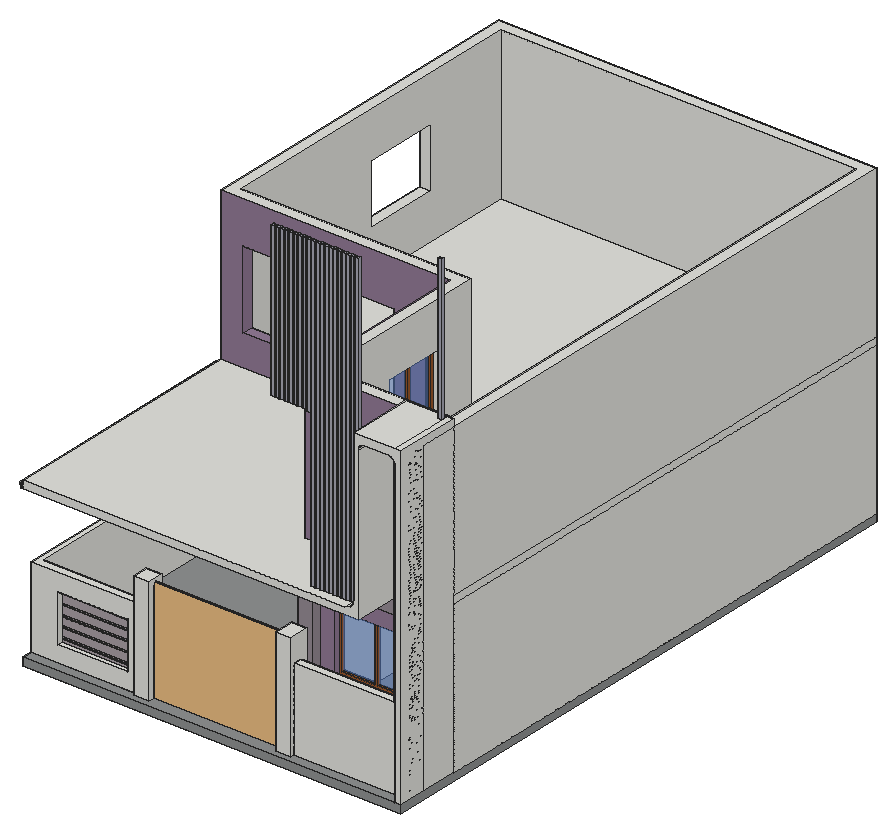
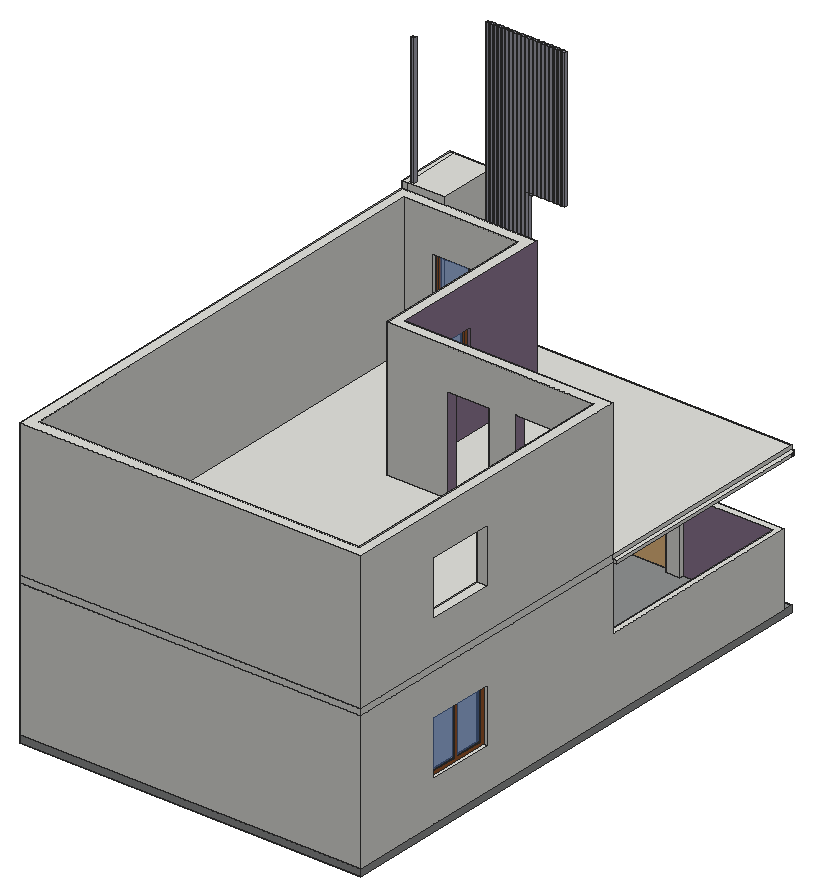
# SketchUp Ruby script. Lengths in inches.
U = 1.inch
M = Sketchup.active_model
def pt(a) = Geom::Point3d.new(a.map { |v| v * U })
def face(e, loops, mat)
  f = e.add_face(loops[0].map { |a| pt(a) })
  loops[1..].each { |l| e.add_face(l.map { |a| pt(a) }).erase! }
  f.material = f.back_material = mat if mat
  f
end
# faces: each face lists its corners as indices into pts; further lists are holes
def faces(e, pts, list, mat = nil) = list.each { |f| face(e, (f[0].is_a?(Array) ? f : [f]).map { |l| l.map { |i| pts[i] } }, mat) }
# xy, xz, yz: faces in a plane at the given z, y or x. An outline is a flat list of corners, or four numbers for a rectangle; further outlines are holes
def ring(l) = l.size == 4 ? [[l[0], l[1]], [l[2], l[1]], [l[2], l[3]], [l[0], l[3]]] : l.each_slice(2).to_a
def flat(e, list, mat, &to3) = list.each { |f| face(e, (f[0].is_a?(Array) ? f : [f]).map { |l| ring(l).map { |u, v| to3.(u, v) } }, mat) }
def xy(e, z, list, mat = nil) = flat(e, list, mat) { |x, y| [x, y, z] }
def xz(e, y, list, mat = nil) = flat(e, list, mat) { |x, z| [x, y, z] }
def yz(e, x, list, mat = nil) = flat(e, list, mat) { |y, z| [x, y, z] }
def lines(e, pts, list) = list.each { |a, b| e.add_line(pt(pts[a]), pt(pts[b])) }
# prism: a flat outline (further loops are holes) pulled along v
def prism(e, loops, v, mat = nil)
  f = face(e, loops, mat); d = Geom::Vector3d.new(v.map { |x| x * U })
  f.pushpull(f.normal.samedirection?(d) ? d.length : -d.length)
end
def box(e, o, s, mat = nil) = prism(e, [[o, [o[0] + s[0], o[1], o[2]], [o[0] + s[0], o[1] + s[1], o[2]], [o[0], o[1] + s[1], o[2]]]], [0, 0, s[2]], mat)
def at(x, y, z, deg = 0) = Geom::Transformation.translation(pt([x, y, z])) * Geom::Transformation.rotation(ORIGIN, Z_AXIS, deg.degrees)
def axes(o, x, y, z) = Geom::Transformation.new([*x, 0, *y, 0, *z, 0, *pt(o).to_a, 1])
def part(name) = M.definitions.add(name)
# library, detail: a bought-in or finely detailed component or shape, given as its bounding box
def library(name, o, s) = part(name).tap { |d| box(d.entities, o, s) }
def detail(e, o, s) = box(e.add_group.entities, o, s)
def put(e, d, t, mat = nil) = e.add_instance(d, t).tap { |i| i.material = mat if mat }
def group(e, t, mat = nil) = e.add_group.tap { |g| g.transformation = t; g.material = mat if mat }.entities
root = M.entities
M.materials.add("0300 AP 7184 STILL POND").color = [167, 167, 180]
M.materials.add("1349 AP 9111 FRESH ORCHID").color = [145, 122, 149]
M.materials.add("1372 AP K056 Arctic Mauve-N").color = [168, 159, 165]
M.materials.add("1373 AP K057 Mauve Meditation-N").color = [149, 139, 148]
M.materials.add("[Blacktop Old 02]").color = [143, 145, 145]
M.materials.add("[Translucent Glass Blue]").color = [100, 149, 237]
M.materials["[Translucent Glass Blue]"].alpha = 0.5
M.materials.add("[Wood Cherry Original]").color = [152, 86, 42]
c1 = library("Untitled",[0,0,0],[36,4.39,84])
c2 = library("Modern Gate 1",[0,0,0],[118.11,1.97,78.74])
c3 = part("Group\#20")
box(c3.entities,[0,0,0],[3.0625,2.375,246])
c4 = part("Group\#10")
box(c4.entities,[0,0,124.49],[3.0625,2.375,121.51])
c5 = part("Group\#19")
xy(c5.entities,0.11,[[0,0,3.0625,2.375]])
xy(c5.entities,246,[[0,0,3.0625,2.375]])
xz(c5.entities,0,[[0,0.11,3.0625,246]])
xz(c5.entities,2.375,[[0,0.11,3.0625,124.49],[0,124.49,3.0625,246]])
yz(c5.entities,0,[[0,0.11,2.375,124.49],[0,124.49,2.375,246]])
yz(c5.entities,3.0625,[[0,0.11,2.375,246]])
c6 = part("Group10\#2")
xy(c6.entities,0,[[-21.5,-21.5,-1.25,21.5],[1.25,-21.5,21.5,21.5]])
c7 = part("Group9\#1")
prism(c7.entities,[[[24,-24,0],[-24,-24,0],[-24,24,0],[24,24,0]],[[-1.25,21.5,0],[-21.5,21.5,0],[-21.5,-21.5,0],[-1.25,-21.5,0]],[[1.25,-21.5,0],[21.5,-21.5,0],[21.5,21.5,0],[1.25,21.5,0]]],[0,0,2])
put(c7.entities,c6,at(0,0,1),"[Translucent Glass Blue]")
c8 = part("Group12\#2")
xy(c8.entities,0,[[-27.5,-21.5,-1.25,21.5],[1.25,-21.5,27.5,21.5]])
c9 = part("Group11\#2")
prism(c9.entities,[[[-30,24,0],[30,24,0],[30,-24,0],[-30,-24,0]],[[1.25,21.5,0],[1.25,-21.5,0],[27.5,-21.5,0],[27.5,21.5,0]],[[-1.25,-21.5,0],[-1.25,21.5,0],[-27.5,21.5,0],[-27.5,-21.5,0]]],[0,0,2])
put(c9.entities,c8,at(0,0,1),"[Translucent Glass Blue]")
c10 = part("Group9\#2")
prism(c10.entities,[[[24,-24,0],[-24,-24,0],[-24,24,0],[24,24,0]],[[-1.25,21.5,0],[-21.5,21.5,0],[-21.5,-21.5,0],[-1.25,-21.5,0]],[[1.25,-21.5,0],[21.5,-21.5,0],[21.5,21.5,0],[1.25,21.5,0]]],[0,0,2])
put(c10.entities,c6,at(0,0,1),"[Translucent Glass Blue]")
c11 = part("Group11\#1")
prism(c11.entities,[[[-30,24,0],[30,24,0],[30,-24,0],[-30,-24,0]],[[1.25,21.5,0],[1.25,-21.5,0],[27.5,-21.5,0],[27.5,21.5,0]],[[-1.25,-21.5,0],[-1.25,21.5,0],[-27.5,21.5,0],[-27.5,-21.5,0]]],[0,0,2])
put(c11.entities,c8,at(0,0,1),"[Translucent Glass Blue]")
c12 = part("Group63\#2")
xy(c12.entities,0,[[-26.0625,-26.25,-9.48,26.25],[-8.29,-26.25,8.29,26.25],[9.48,-26.25,26.0625,26.25]])
c13 = part("Group62\#1")
prism(c13.entities,[[[-30,-30.1875,0],[-30,30.1875,0],[30,30.1875,0],[30,-30.1875,0]],[[-9.48,26.25,0],[-26.0625,26.25,0],[-26.0625,-26.25,0],[-9.48,-26.25,0]],[[9.48,26.25,0],[9.48,-26.25,0],[26.0625,-26.25,0],[26.0625,26.25,0]],[[-8.29,26.25,0],[-8.29,-26.25,0],[8.29,-26.25,0],[8.29,26.25,0]]],[0,0,5.875])
put(c13.entities,c12,at(0,0,2.9375),"[Translucent Glass Blue]")
c14 = part("Group4\#2")
xy(c14.entities,0,[[-27.5,-21.5,-1.25,21.5],[1.25,-21.5,27.5,21.5]])
c15 = part("Group3\#1")
prism(c15.entities,[[[30,24,0],[30,-24,0],[-30,-24,0],[-30,24,0]],[[27.5,-21.5,0],[27.5,21.5,0],[1.25,21.5,0],[1.25,-21.5,0]],[[-27.5,21.5,0],[-27.5,-21.5,0],[-1.25,-21.5,0],[-1.25,21.5,0]]],[0,0,2])
put(c15.entities,c14,at(0,0,1),"[Translucent Glass Blue]")
g1 = group(root,at(21.875,58.1875,-6),"[Blacktop Old 02]")
box(g1,[0,-52.5625,0],[300,472.5625,6])
put(root,c1,at(123.5625,204.4,0))
put(root,c2,axes([117.75,16.2,0],[0.83803,0,0],[0,1,0],[0,0,1.0465]))
g2 = group(root,at(21.875,58.1875,120))
xy(g2,-120,[[295.5,-52.5625,300,-29.9375]])
xy(g2,0,[[0.83,-52.5625,-0.63,-52.43,-1.82,-52.03,-2.75,-51.37,-3.41,-50.44,-3.81,-49.25,-3.9375,-47.8,-3.9375,144.125,0,144.125,0,420,300,420,300,0,266.53,0,266.53,-52.5625]])
xy(g2,3,[[0,-52.5625,0,144.125,-3.9375,144.125,-3.9375,-47.8,-3.83,-49.25,-3.5,-50.44,-2.95,-51.37,-2.1875,-52.03,-1.2,-52.43]])
xy(g2,6,[[0,-52.5625,255.76,-52.5625,255.76,0,300,0,300,420,0,420]])
xy(g2,126,[[271.39,-52.5625,271.39,0,295.5,0,295.5,-29.9375,288.53,-29.9375,288.53,-52.5625],[295.5,-29.9375,300,0]])
xy(g2,132,[[262.58,-52.5625,295.5,0],[295.5,-52.5625,300,0]])
xz(g2,-52.5625,[[295.5,-120,300,-120,300,132,262.58,132,262.58,12.82,262.39,10.74,261.82,9.03,260.875,7.7,259.55,6.76,257.84,6.1875,255.76,6,0,6,0,3,0.83,0,266.53,0,266.53,121.14,266.67,122.625,267.07,123.84,267.75,124.78,268.69,125.46,269.91,125.86,271.39,126,288.53,126,290.66,125.81,292.4,125.23,293.76,124.26,294.73,122.9,295.31,121.16,295.5,119.03]])
xz(g2,-29.9375,[[295.5,-120,295.5,119.03,295.31,121.16,294.73,122.9,293.76,124.26,292.4,125.23,290.66,125.81,288.53,126,300,126,300,-120]])
xz(g2,0,[[266.53,0,300,6],[255.76,6,257.84,6.1875,259.55,6.76,260.875,7.7,261.82,9.03,262.39,10.74,262.58,12.82,262.58,132,295.5,132,295.5,126,271.39,126,269.91,125.86,268.69,125.46,267.75,124.78,267.07,123.84,266.67,122.625,266.53,121.14,266.53,6],[295.5,126,300,132]])
xz(g2,144.125,[[-3.9375,0,0,3]])
xz(g2,420,[[0,0,300,6]])
yz(g2,-3.9375,[[-47.8,0,144.125,3]])
yz(g2,0,[[144.125,0,420,6],[-52.5625,3,144.125,6]])
yz(g2,262.58,[[-52.5625,12.82,0,132]])
yz(g2,266.53,[[-52.5625,0,0,121.14]])
yz(g2,295.5,[[-52.5625,-120,-29.9375,119.03]])
yz(g2,300,[[-52.5625,-120,-29.9375,-120,-29.9375,126,0,126,0,132,-52.5625,132],[0,0,420,6]])
p = [[-0.63,-52.43,0],[0.83,-52.5625,0],[-1.2,-52.43,3],[0,-52.5625,3],[-2.1875,-52.03,3],[-1.82,-52.03,0],
  [-2.95,-51.37,3],[-2.75,-51.37,0],[-3.5,-50.44,3],[-3.41,-50.44,0],[-3.81,-49.25,0],[-3.83,-49.25,3],
  [-3.9375,-47.8,3],[-3.9375,-47.8,0],[257.84,-52.5625,6.1875],[257.84,0,6.1875],[255.76,0,6],[255.76,-52.5625,6],
  [259.55,-52.5625,6.76],[259.55,0,6.76],[260.875,-52.5625,7.7],[260.875,0,7.7],[261.82,-52.5625,9.03],[261.82,0,9.03],
  [262.39,-52.5625,10.74],[262.39,0,10.74],[262.58,-52.5625,12.82],[262.58,0,12.82],[295.31,-52.5625,121.16],[295.31,-29.9375,121.16],
  [295.5,-29.9375,119.03],[295.5,-52.5625,119.03],[266.67,0,122.625],[266.67,-52.5625,122.625],[266.53,-52.5625,121.14],[266.53,0,121.14],
  [294.73,-52.5625,122.9],[294.73,-29.9375,122.9],[267.07,0,123.84],[267.07,-52.5625,123.84],[293.76,-52.5625,124.26],[293.76,-29.9375,124.26],
  [267.75,0,124.78],[267.75,-52.5625,124.78],[292.4,-52.5625,125.23],[292.4,-29.9375,125.23],[268.69,0,125.46],[268.69,-52.5625,125.46],
  [290.66,-52.5625,125.81],[290.66,-29.9375,125.81],[269.91,0,125.86],[269.91,-52.5625,125.86],[288.53,-52.5625,126],[288.53,-29.9375,126],
  [271.39,0,126],[271.39,-52.5625,126]]
faces(g2,p,[[0,1,2],[1,3,2],[0,2,4],[5,0,4],[5,4,6],[7,5,6],[7,6,8],[9,7,8],
  [10,9,11],[9,8,11],[10,11,12],[13,10,12],[14,15,16,17],[18,19,15,14],[20,21,19,18],[22,23,21,20],
  [24,25,23,22],[26,27,25,24],[28,29,30,31],[32,33,34,35],[36,37,29,28],[38,39,33,32],[40,41,37,36],[42,43,39,38],
  [44,45,41,40],[46,47,43,42],[48,49,45,44],[50,51,47,46],[52,53,49,48],[54,55,51,50]])
put(g2,c3,at(226.96,-45.3125,6),"0300 AP 7184 STILL POND")
g3 = group(g2,at(230.4,-45.3125,6),"0300 AP 7184 STILL POND")
box(g3,[0,0,0],[3.0625,2.375,246])
put(g2,c3,at(233.84,-45.3125,6),"0300 AP 7184 STILL POND")
put(g2,c3,at(237.28,-45.3125,6),"0300 AP 7184 STILL POND")
put(g2,c3,at(240.71,-45.3125,6),"0300 AP 7184 STILL POND")
put(g2,c3,at(244.15,-45.3125,6),"0300 AP 7184 STILL POND")
put(g2,c3,at(247.59,-45.3125,6),"0300 AP 7184 STILL POND")
put(g2,c3,at(251.03,-45.3125,6),"0300 AP 7184 STILL POND")
put(g2,c3,at(254.46,-45.3125,6),"0300 AP 7184 STILL POND")
put(g2,c3,at(257.9,-45.3125,6),"0300 AP 7184 STILL POND")
put(g2,c4,at(191.3125,-45.3125,6),"0300 AP 7184 STILL POND")
put(g2,c4,at(194.89,-45.3125,6),"0300 AP 7184 STILL POND")
put(g2,c4,at(198.46,-45.3125,6),"0300 AP 7184 STILL POND")
put(g2,c4,at(202.04,-45.3125,6),"0300 AP 7184 STILL POND")
put(g2,c4,at(205.61,-45.3125,6),"0300 AP 7184 STILL POND")
put(g2,c4,at(209.1875,-45.3125,6),"0300 AP 7184 STILL POND")
put(g2,c4,at(212.76,-45.3125,6),"0300 AP 7184 STILL POND")
put(g2,c4,at(216.33,-45.3125,6),"0300 AP 7184 STILL POND")
g4 = group(g2,at(219.96,-45.3125,6),"0300 AP 7184 STILL POND")
xy(g4,123.23,[[0,0,3.0625,2.375]])
xy(g4,246,[[0,0,3.0625,2.375]])
xz(g4,0,[[0,123.23,3.0625,246]])
xz(g4,2.375,[[0,123.23,3.0625,124.49],[0,124.49,3.0625,246]])
yz(g4,0,[[0,123.23,2.375,124.49],[0,124.49,2.375,246]])
yz(g4,3.0625,[[0,123.23,2.375,246]])
put(g2,c5,at(223.24,-45.3125,5.89),"0300 AP 7184 STILL POND")
g5 = group(g2,at(267.59,-5.2,-0.11),"0300 AP 7184 STILL POND")
xy(g5,0.11,[[0,0,3.0625,2.375]])
xy(g5,126.11,[[0,0,3.0625,2.375]])
xz(g5,0,[[0,0.11,3.0625,126.11]])
xz(g5,2.375,[[0,0.11,3.0625,124.49],[0,124.49,3.0625,126.11]])
yz(g5,0,[[0,0.11,2.375,124.49],[0,124.49,2.375,126.11]])
yz(g5,3.0625,[[0,0.11,2.375,126.11]])
g6 = group(g2,at(271.03,-5.2,-0.11),"0300 AP 7184 STILL POND")
xy(g6,0.11,[[0,0,3.0625,2.375]])
xy(g6,126.11,[[0,0,3.0625,2.375]])
xz(g6,0,[[0,0.11,3.0625,126.11]])
xz(g6,2.375,[[0,0.11,3.0625,124.49],[0,124.49,3.0625,126.11]])
yz(g6,0,[[0,0.11,2.375,124.49],[0,124.49,2.375,126.11]])
yz(g6,3.0625,[[0,0.11,2.375,126.11]])
g7 = group(g2,at(274.48,-5.2,-0.11),"0300 AP 7184 STILL POND")
xy(g7,0.11,[[0,0,3.0625,2.375]])
xy(g7,126.11,[[0,0,3.0625,2.375]])
xz(g7,0,[[0,0.11,3.0625,126.11]])
xz(g7,2.375,[[0,0.11,3.0625,124.49],[0,124.49,3.0625,126.11]])
yz(g7,0,[[0,0.11,2.375,124.49],[0,124.49,2.375,126.11]])
yz(g7,3.0625,[[0,0.11,2.375,126.11]])
g8 = group(g2,at(277.93,-5.2,-0.11),"0300 AP 7184 STILL POND")
xy(g8,0.11,[[0,0,3.0625,2.375]])
xy(g8,130.6875,[[0,0,3.0625,2.375]])
xz(g8,0,[[0,0.11,3.0625,130.6875]])
xz(g8,2.375,[[0,0.11,3.0625,124.49],[0,124.49,3.0625,130.6875]])
yz(g8,0,[[0,0.11,2.375,124.49],[0,124.49,2.375,130.6875]])
yz(g8,3.0625,[[0,0.11,2.375,130.6875]])
g9 = group(g2,at(281.37,-5.2,-0.11),"0300 AP 7184 STILL POND")
xy(g9,0.11,[[0,0,3.0625,2.375]])
xy(g9,126.01,[[0,0,3.0625,2.375]])
xz(g9,0,[[0,0.11,3.0625,126.01]])
xz(g9,2.375,[[0,0.11,3.0625,124.49],[0,124.49,3.0625,126.01]])
yz(g9,0,[[0,0.11,2.375,124.49],[0,124.49,2.375,126.01]])
yz(g9,3.0625,[[0,0.11,2.375,126.01]])
g10 = group(g2,at(284.82,-5.2,-0.11),"0300 AP 7184 STILL POND")
xy(g10,0.11,[[0,0,3.0625,2.375]])
xy(g10,126.01,[[0,0,3.0625,2.375]])
xz(g10,0,[[0,0.11,3.0625,126.01]])
xz(g10,2.375,[[0,0.11,3.0625,124.49],[0,124.49,3.0625,126.01]])
yz(g10,0,[[0,0.11,2.375,124.49],[0,124.49,2.375,126.01]])
yz(g10,3.0625,[[0,0.11,2.375,126.01]])
g11 = group(g2,at(288.27,-5.2,-0.11),"0300 AP 7184 STILL POND")
xy(g11,0.11,[[0,0,3.0625,2.375]])
xy(g11,126.01,[[0,0,3.0625,2.375]])
xz(g11,0,[[0,0.11,3.0625,126.01]])
xz(g11,2.375,[[0,0.11,3.0625,124.49],[0,124.49,3.0625,126.01]])
yz(g11,0,[[0,0.11,2.375,124.49],[0,124.49,2.375,126.01]])
yz(g11,3.0625,[[0,0.11,2.375,126.01]])
put(g2,c5,at(291.71,-5.2,-0.11),"0300 AP 7184 STILL POND")
g12 = group(root,at(21.875,58.1875,126))
xy(g12,-126,[[196.875,-47.1875,208.875,-31.8125],[208.875,-44.1875,208.875,-37.8125,295,-37.8125,295,-25.4375,300,-25.4375,300,-44.1875],[295,-25.4375,300,0]])
xy(g12,-60.49,[[208.875,-44.1875,288.125,-37.8125]])
xy(g12,-41.05,[[196.875,-47.1875,208.875,-31.8125]])
xy(g12,0,[[182.15,0,182.15,144.125,137.6875,144.125,137.6875,153.125,191.15,153.125,191.15,9,291,9,291,411,9,411,9,153.125,101.6875,153.125,101.6875,144.125,0,144.125,0,420,300,420,300,0]])
xy(g12,24.375,[[17.6875,144.125,77.6875,153.125]],"1349 AP 9111 FRESH ORCHID")
xy(g12,36,[[206.15,4.5,266.15,9],[186.65,72.125,191.15,120.125],[0,281.375,9,341.375]])
xy(g12,36,[[206.15,0,266.15,4.5],[182.15,72.125,186.65,120.125]],"1349 AP 9111 FRESH ORCHID")
xy(g12,84,[[206.15,4.5,266.15,9],[186.65,72.125,191.15,120.125],[0,281.375,9,341.375]])
xy(g12,84,[[206.15,0,266.15,4.5],[182.15,72.125,186.65,120.125],[101.6875,144.125,137.6875,153.125]],"1349 AP 9111 FRESH ORCHID")
xy(g12,86.75,[[17.6875,144.125,77.6875,153.125]],"1349 AP 9111 FRESH ORCHID")
xy(g12,120,[[288.125,-44.1875,300,-44.1875,300,-25.4375,295,-25.4375,295,-37.8125,288.125,-37.8125],[295,-25.4375,300,0],[[182.15,0,300,0,300,420,0,420,0,144.125,182.15,144.125],[191.15,9,191.15,153.125,9,153.125,9,411,291,411,291,9]]])
xz(g12,-47.1875,[[196.875,-126,208.875,-41.05]])
xz(g12,-44.1875,[[208.875,-126,300,-126,300,120,288.125,120,288.125,-60.49,208.875,-60.49]])
xz(g12,-37.8125,[[208.875,-126,208.875,-60.49,288.125,-60.49,288.125,120,295,120,295,-126]])
xz(g12,-31.8125,[[196.875,-126,208.875,-41.05]])
xz(g12,0,[[295,-126,300,0],[295,0,300,120]])
xz(g12,0,[[[182.15,0,295,120],[206.15,36,266.15,84]]],"1349 AP 9111 FRESH ORCHID")
xz(g12,9,[[[191.15,0,291,120],[206.15,36,266.15,84]]])
xz(g12,72.125,[[186.65,36,191.15,84]])
xz(g12,72.125,[[182.15,36,186.65,84]],"1349 AP 9111 FRESH ORCHID")
xz(g12,120.125,[[186.65,36,191.15,84]])
xz(g12,120.125,[[182.15,36,186.65,84]],"1349 AP 9111 FRESH ORCHID")
xz(g12,144.125,[[[0,0,101.6875,0,101.6875,84,137.6875,84,137.6875,0,182.15,0,182.15,120,0,120],[17.6875,24.375,77.6875,86.75]]],"1349 AP 9111 FRESH ORCHID")
xz(g12,153.125,[[[9,0,9,120,191.15,120,191.15,0,137.6875,0,137.6875,84,101.6875,84,101.6875,0],[17.6875,24.375,77.6875,86.75]]])
xz(g12,281.375,[[0,36,9,84]])
xz(g12,341.375,[[0,36,9,84]])
xz(g12,411,[[9,0,291,120]])
xz(g12,420,[[0,0,300,120]])
yz(g12,0,[[[144.125,0,420,120],[281.375,36,341.375,84]]])
yz(g12,9,[[[153.125,0,411,120],[281.375,36,341.375,84]]])
yz(g12,17.6875,[[144.125,24.375,153.125,86.75]],"1349 AP 9111 FRESH ORCHID")
yz(g12,77.6875,[[144.125,24.375,153.125,86.75]],"1349 AP 9111 FRESH ORCHID")
yz(g12,101.6875,[[144.125,0,153.125,84]],"1349 AP 9111 FRESH ORCHID")
yz(g12,137.6875,[[144.125,0,153.125,84]],"1349 AP 9111 FRESH ORCHID")
yz(g12,182.15,[[[0,0,144.125,120],[72.125,36,120.125,84]]],"1349 AP 9111 FRESH ORCHID")
yz(g12,191.15,[[[9,0,153.125,120],[72.125,36,120.125,84]]])
yz(g12,196.875,[[-47.1875,-126,-31.8125,-41.05]])
yz(g12,206.15,[[4.5,36,9,84]])
yz(g12,206.15,[[0,36,4.5,84]],"1349 AP 9111 FRESH ORCHID")
yz(g12,208.875,[[-47.1875,-126,-44.1875,-126,-44.1875,-60.49,-37.8125,-60.49,-37.8125,-126,-31.8125,-126,-31.8125,-41.05,-47.1875,-41.05],[-44.1875,-126,-37.8125,-60.49]])
yz(g12,266.15,[[4.5,36,9,84]])
yz(g12,266.15,[[0,36,4.5,84]],"1349 AP 9111 FRESH ORCHID")
yz(g12,288.125,[[-44.1875,-60.49,-37.8125,120]])
yz(g12,291,[[9,0,411,120]])
yz(g12,295,[[-37.8125,-126,0,120]])
yz(g12,300,[[-44.1875,-126,0,120],[0,0,420,120]])
put(g12,c7,axes([187.65,96.125,60],[0,-1,0],[0,0,1],[-1,0,0]),"[Wood Cherry Original]")
put(g12,c9,axes([236.15,3.5,60],[-1,0,0],[0,0,1],[0,1,0]),"[Wood Cherry Original]")
g13 = group(root,at(21.875,58.1875,0))
xy(g13,0,[[83.875,-47.1875,95.875,-34.8125],[0,-44.1875,83.875,-37.8125],[0,-37.8125,0,420,300,420,300,0,182.15,0,182.15,144.125,137.6875,144.125,137.6875,153.125,191.15,153.125,191.15,9,291,9,291,411,9,411,9,153.125,101.6875,153.125,101.6875,144.125,4.5,144.125,4.5,-37.8125]])
xy(g13,12.64,[[21.17,-44.1875,76.73,-40.3125]])
xy(g13,15.05,[[21.17,-40.3125,76.73,-39.3125]])
xy(g13,16.99,[[21.17,-40.3125,76.73,-39.3125]])
xy(g13,23.05,[[21.17,-40.3125,76.73,-39.3125]])
xy(g13,23.625,[[17.6875,148.625,77.6875,153.125]])
xy(g13,23.625,[[17.6875,144.125,77.6875,148.625]],"1349 AP 9111 FRESH ORCHID")
xy(g13,24.99,[[21.17,-40.3125,76.73,-39.3125]])
xy(g13,31.05,[[21.17,-40.3125,76.73,-39.3125]])
xy(g13,32.99,[[21.17,-40.3125,76.73,-39.3125]])
xy(g13,36,[[0,281.375,4.5,341.375],[4.5,281.375,9,341.375]])
xy(g13,36,[[206.15,0,266.15,4.5],[206.15,4.5,266.15,9],[182.15,72.125,186.65,120.125],[186.65,72.125,191.15,120.125]],"1349 AP 9111 FRESH ORCHID")
xy(g13,39.05,[[21.17,-40.3125,76.73,-39.3125]])
xy(g13,40.99,[[21.17,-40.3125,76.73,-39.3125]])
xy(g13,47.05,[[21.17,-40.3125,76.73,-39.3125]])
xy(g13,48.99,[[21.17,-40.3125,76.73,-39.3125]])
xy(g13,50.58,[[21.17,-44.1875,76.73,-40.3125]])
xy(g13,64.1875,[[0,-44.1875,83.875,-44.1875,83.875,-37.8125,4.5,-37.8125,4.5,144.125,0,144.125]])
xy(g13,84,[[101.6875,144.125,137.6875,153.125],[17.6875,148.625,77.6875,153.125],[0,281.375,4.5,341.375],[4.5,281.375,9,341.375]])
xy(g13,84,[[206.15,0,266.15,4.5],[206.15,4.5,266.15,9],[182.15,72.125,186.65,120.125],[186.65,72.125,191.15,120.125],[17.6875,144.125,77.6875,148.625]],"1349 AP 9111 FRESH ORCHID")
xy(g13,84.95,[[83.875,-47.1875,95.875,-34.8125]])
xy(g13,120,[[[182.15,0,300,0,300,420,0,420,0,144.125,182.15,144.125],[191.15,9,191.15,153.125,9,153.125,9,411,291,411,291,9]]])
xz(g13,-47.1875,[[83.875,0,95.875,84.95]])
xz(g13,-44.1875,[[[0,0,83.875,64.1875],[21.17,12.64,76.73,50.58]]])
xz(g13,-40.3125,[[21.17,12.64,76.73,15.05],[21.17,16.99,76.73,23.05],[21.17,24.99,76.73,31.05],[21.17,32.99,76.73,39.05],[21.17,40.99,76.73,47.05],
  [21.17,48.99,76.73,50.58]],"1372 AP K056 Arctic Mauve-N")
xz(g13,-39.3125,[[21.17,15.05,76.73,16.99],[21.17,23.05,76.73,24.99],[21.17,31.05,76.73,32.99],[21.17,39.05,76.73,40.99],[21.17,47.05,76.73,48.99]],"1372 AP K056 Arctic Mauve-N")
xz(g13,-37.8125,[[4.5,0,83.875,64.1875]],"1349 AP 9111 FRESH ORCHID")
xz(g13,-34.8125,[[83.875,0,95.875,84.95]])
xz(g13,0,[[[194.03,0,300,0,300,120,282.04,120,282.04,101.0625,194.03,101.0625],[206.15,36,266.15,84]]],"1349 AP 9111 FRESH ORCHID")
xz(g13,9,[[[191.15,0,291,120],[206.15,36,266.15,84]]])
xz(g13,72.125,[[182.15,36,186.65,84],[186.65,36,191.15,84]],"1349 AP 9111 FRESH ORCHID")
xz(g13,120.125,[[182.15,36,186.65,84],[186.65,36,191.15,84]],"1349 AP 9111 FRESH ORCHID")
xz(g13,144.125,[[[4.5,0,101.6875,0,101.6875,84,137.6875,84,137.6875,0,182.15,0,182.15,120,0,120,0,64.1875,4.5,64.1875],[17.6875,23.625,77.6875,84]]],"1349 AP 9111 FRESH ORCHID")
xz(g13,153.125,[[[9,0,9,120,191.15,120,191.15,0,137.6875,0,137.6875,84,101.6875,84,101.6875,0],[17.6875,23.625,77.6875,84]]])
xz(g13,281.375,[[0,36,4.5,84],[4.5,36,9,84]])
xz(g13,341.375,[[0,36,4.5,84],[4.5,36,9,84]])
xz(g13,411,[[9,0,291,120]])
xz(g13,420,[[0,0,300,120]])
yz(g13,0,[[[-44.1875,0,-44.1875,64.1875,144.125,64.1875,144.125,120,420,120,420,0],[281.375,36,341.375,84]]])
yz(g13,4.5,[[-37.8125,0,144.125,64.1875]])
yz(g13,9,[[[153.125,0,411,120],[281.375,36,341.375,84]]])
yz(g13,17.6875,[[148.625,23.625,153.125,84]])
yz(g13,17.6875,[[144.125,23.625,148.625,84]],"1349 AP 9111 FRESH ORCHID")
yz(g13,21.17,[[-44.1875,12.64,-40.3125,50.58]])
yz(g13,76.73,[[-44.1875,12.64,-40.3125,50.58]])
yz(g13,77.6875,[[148.625,23.625,153.125,84]])
yz(g13,77.6875,[[144.125,23.625,148.625,84]],"1349 AP 9111 FRESH ORCHID")
yz(g13,83.875,[[-47.1875,0,-47.1875,84.95,-34.8125,84.95,-34.8125,0,-37.8125,0,-37.8125,64.1875,-44.1875,64.1875,-44.1875,0],[-44.1875,0,-37.8125,64.1875]])
yz(g13,95.875,[[-47.1875,0,-34.8125,84.95]])
yz(g13,101.6875,[[144.125,0,153.125,84]],"1349 AP 9111 FRESH ORCHID")
yz(g13,137.6875,[[144.125,0,153.125,84]],"1349 AP 9111 FRESH ORCHID")
yz(g13,182.15,[[[0,0,144.125,120],[72.125,36,120.125,84]]],"1349 AP 9111 FRESH ORCHID")
yz(g13,191.15,[[[9,0,153.125,120],[72.125,36,120.125,84]]])
yz(g13,206.15,[[0,36,4.5,84],[4.5,36,9,84]],"1349 AP 9111 FRESH ORCHID")
yz(g13,266.15,[[0,36,4.5,84],[4.5,36,9,84]],"1349 AP 9111 FRESH ORCHID")
yz(g13,291,[[9,0,411,120]])
yz(g13,300,[[0,0,420,120]])
put(g13,c10,axes([187.65,96.125,60],[0,-1,0],[0,0,1],[-1,0,0]),"[Wood Cherry Original]")
put(g13,c11,axes([236.15,3.5,60],[-1,0,0],[0,0,1],[0,1,0]),"[Wood Cherry Original]")
g14 = group(g13,at(182.15,0,0))
xy(g14,0,[[0,-7.5,11.88,0]])
xy(g14,101.0625,[[11.88,-7.5,112.85,0]],"1373 AP K057 Mauve Meditation-N")
xy(g14,120,[[0,-7.5,112.85,0]])
xz(g14,-7.5,[[0,0,11.88,0,11.88,101.0625,112.85,101.0625,112.85,120,0,120]],"1373 AP K057 Mauve Meditation-N")
xz(g14,0,[[0,0,0,120,112.85,120,112.85,101.0625,11.88,101.0625,11.88,0]])
yz(g14,0,[[-7.5,0,0,120]],"1373 AP K057 Mauve Meditation-N")
yz(g14,11.88,[[-7.5,0,0,101.0625]],"1373 AP K057 Mauve Meditation-N")
yz(g14,112.85,[[-7.5,101.0625,0,120]])
put(g13,c13,axes([47.6875,145.6875,53.8125],[-1,0,0],[0,0,1],[0,1,0]),"[Wood Cherry Original]")
put(root,c15,axes([27.375,369.5625,60],[0,-1,0],[0,0,1],[-1,0,0]),"[Wood Cherry Original]")
